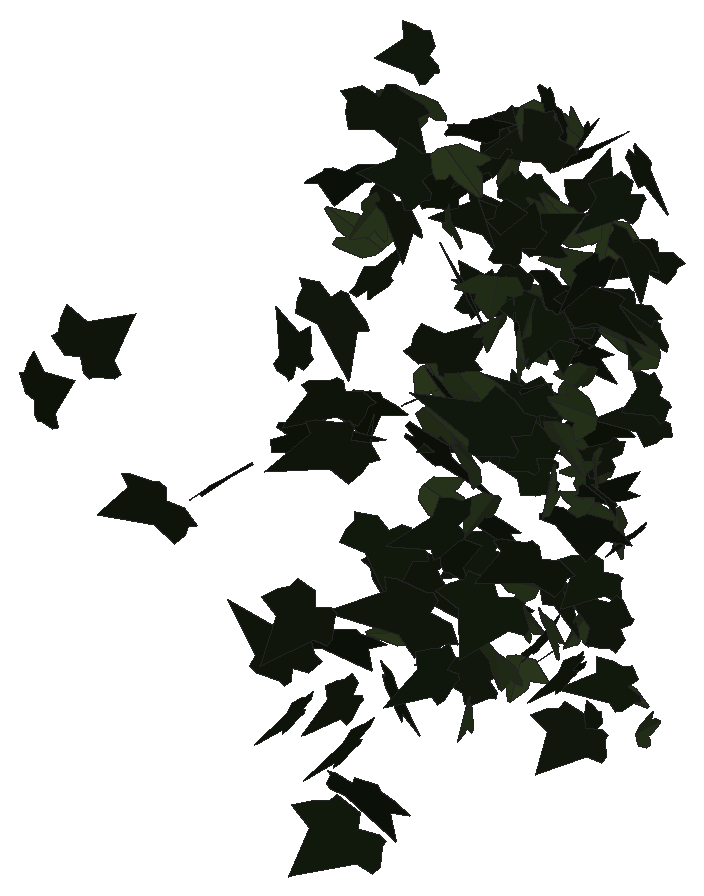
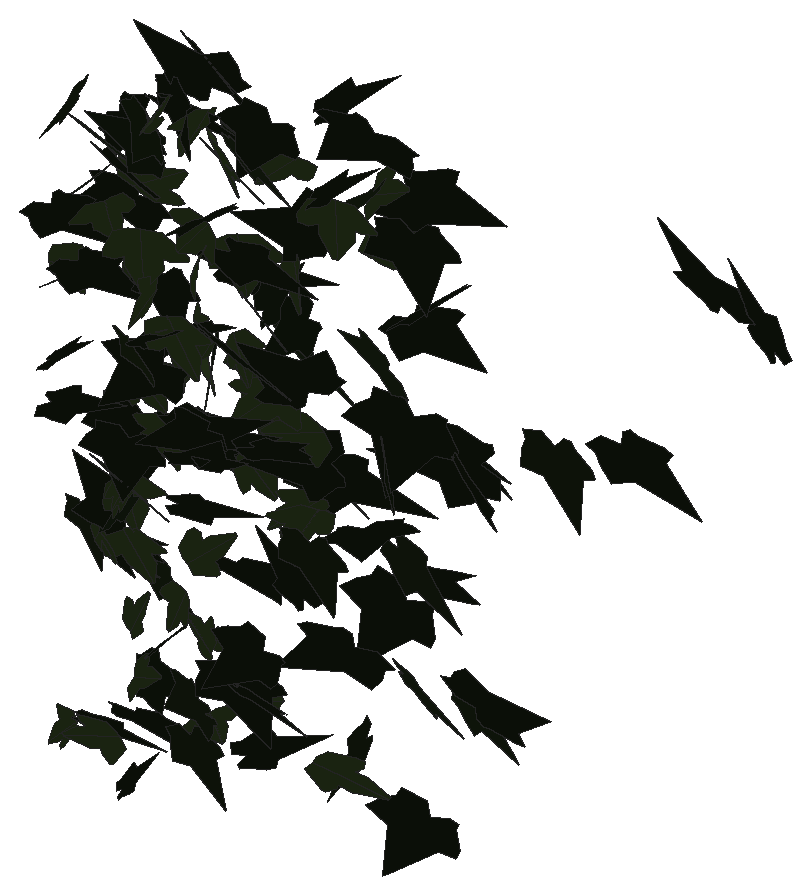
# SketchUp Ruby script. Lengths in inches.
U = 1.inch
M = Sketchup.active_model
def pt(a) = Geom::Point3d.new(a.map { |v| v * U })
def face(e, loops, mat)
  f = e.add_face(loops[0].map { |a| pt(a) })
  loops[1..].each { |l| e.add_face(l.map { |a| pt(a) }).erase! }
  f.material = f.back_material = mat if mat
  f
end
# faces: each face lists its corners as indices into pts; further lists are holes
def faces(e, pts, list, mat = nil) = list.each { |f| face(e, (f[0].is_a?(Array) ? f : [f]).map { |l| l.map { |i| pts[i] } }, mat) }
# xy, xz, yz: faces in a plane at the given z, y or x. An outline is a flat list of corners, or four numbers for a rectangle; further outlines are holes
def ring(l) = l.size == 4 ? [[l[0], l[1]], [l[2], l[1]], [l[2], l[3]], [l[0], l[3]]] : l.each_slice(2).to_a
def flat(e, list, mat, &to3) = list.each { |f| face(e, (f[0].is_a?(Array) ? f : [f]).map { |l| ring(l).map { |u, v| to3.(u, v) } }, mat) }
def xy(e, z, list, mat = nil) = flat(e, list, mat) { |x, y| [x, y, z] }
def xz(e, y, list, mat = nil) = flat(e, list, mat) { |x, z| [x, y, z] }
def yz(e, x, list, mat = nil) = flat(e, list, mat) { |y, z| [x, y, z] }
def lines(e, pts, list) = list.each { |a, b| e.add_line(pt(pts[a]), pt(pts[b])) }
# prism: a flat outline (further loops are holes) pulled along v
def prism(e, loops, v, mat = nil)
  f = face(e, loops, mat); d = Geom::Vector3d.new(v.map { |x| x * U })
  f.pushpull(f.normal.samedirection?(d) ? d.length : -d.length)
end
def box(e, o, s, mat = nil) = prism(e, [[o, [o[0] + s[0], o[1], o[2]], [o[0] + s[0], o[1] + s[1], o[2]], [o[0], o[1] + s[1], o[2]]]], [0, 0, s[2]], mat)
def at(x, y, z, deg = 0) = Geom::Transformation.translation(pt([x, y, z])) * Geom::Transformation.rotation(ORIGIN, Z_AXIS, deg.degrees)
def axes(o, x, y, z) = Geom::Transformation.new([*x, 0, *y, 0, *z, 0, *pt(o).to_a, 1])
def part(name) = M.definitions.add(name)
# library, detail: a bought-in or finely detailed component or shape, given as its bounding box
def library(name, o, s) = part(name).tap { |d| box(d.entities, o, s) }
def detail(e, o, s) = box(e.add_group.entities, o, s)
def put(e, d, t, mat = nil) = e.add_instance(d, t).tap { |i| i.material = mat if mat }
def group(e, t, mat = nil) = e.add_group.tap { |g| g.transformation = t; g.material = mat if mat }.entities
root = M.entities
M.materials.add("1026 AP 7946 SUNNY SIDE UP").color = [254, 231, 186]
M.materials.add("efeu1").color = [18, 25, 13]
M.materials.add("efeu2").color = [43, 57, 29]
c1 = part("ivyleaf_9")
p = [[1.54,2.16,1.25],[1.36,2.04,1.19],[-0.21,0.99,0.68],[-0.71,1.11,0.82],[-0.85,0.86,0.67],[-0.8,0.17,0.21],
  [-0.9,-0.01,0.1],[-0.67,-0.16,-0.02],[-0.08,-0.08,-0.05],[-0.03,-0.6,-0.4],[0.65,-0.88,-0.66],[0.83,-0.6,-0.49],
  [1.29,-0.42,-0.43],[1.8125,-0.07,-0.26],[1.21,0.44,0.15]]
faces(c1.entities,p,[[0,1,2,3,4,5,6,7,8,9,10,11,12,13,14]],"efeu1")
c2 = part("ivyleaf_10")
p = [[0,0.5,-0.03],[-0.0625,2.02,-0.43],[-0.19,2.01,-0.46],[-0.54,1.05,-0.29],[-0.52,0.625,-0.18],[-0.83,0.76,-0.28],
  [-1.16,0.64,-0.33],[-1.15,0.33,-0.24],[-0.77,-0.39,0.02],[-0.3,-0.51,0.16],[0.04,-0.48,0.23],[-0.02,2.01,-0.4375],
  [-0.06,2.01,-0.43],[0.04,-0.49,0.23],[0.67,-0.49,0.14],[1.38,0.36,-0.2],[1.375,0.51,-0.24],[0.81,0.65,-0.19],
  [0.62,0.59,-0.15],[0.6,1.09,-0.28],[0.5,1.23,-0.31]]
faces(c2.entities,p,[[0,1,2,3,4,5,6,7,8,9,10],[11,12,0,13,14,15,16,17,18,19,20]],"efeu2")
put(root,c1,axes([89.9,204.5625,274.55],[-0.05086,0.1436,0.39421],[0.18993,-0.34913,0.15144],[0.64039,0.11495,-0.01361]),"1026 AP 7946 SUNNY SIDE UP")
put(root,c1,axes([96.67,204.76,268.41],[-0.56224,-0.22577,0.12999],[-0.1429,-0.09664,-0.42919],[0.41356,-0.34033,0.02842]),"1026 AP 7946 SUNNY SIDE UP")
put(root,c1,axes([90.46,205.12,275.36],[-0.2526,0.22111,0.33746],[0.34026,-0.24042,0.2811],[0.55336,0.24877,-0.01881]),"1026 AP 7946 SUNNY SIDE UP")
put(root,c1,axes([95.93,205.48,275.42],[-0.08247,-0.01961,-0.43984],[-0.03894,-0.41267,0.01825],[-0.6967,0.02539,0.05105]),"1026 AP 7946 SUNNY SIDE UP")
put(root,c1,axes([94.96,205.73,271.71],[-0.65961,0.01646,-0.14293],[0.22051,-0.06256,-0.41322],[-0.0607,-0.40614,0.05205]),"1026 AP 7946 SUNNY SIDE UP")
put(root,c1,axes([91.76,205.69,272.69],[0.08639,0.01748,-0.39329],[-0.52238,-0.20149,-0.05868],[-0.34261,0.31163,-0.0097]),"1026 AP 7946 SUNNY SIDE UP")
put(root,c1,axes([95.93,205.72,269.49],[-0.3892,0.29505,-0.15727],[0.12168,-0.13481,-0.40107],[-0.54913,-0.23899,0.02259]),"1026 AP 7946 SUNNY SIDE UP")
put(root,c1,axes([95.94,205.67,268.62],[0.64221,0.04593,-0.10351],[-0.15486,-0.05156,-0.40657],[-0.09679,0.38721,-0.03628]),"1026 AP 7946 SUNNY SIDE UP")
put(root,c1,axes([97.34,206.36,271.05],[-0.56522,0.17945,-0.0836],[0.08926,-0.07116,-0.40401],[-0.32168,-0.33507,0.0348]),"1026 AP 7946 SUNNY SIDE UP")
put(root,c1,axes([92.29,206.66,272.89],[-0.04108,0.37676,-0.00245],[-0.00981,-0.00759,-0.40423],[-0.63961,-0.02408,0.00636]),"1026 AP 7946 SUNNY SIDE UP")
put(root,c1,axes([96.24,207.23,271.41],[-0.13267,-0.09029,-0.43018],[-0.4186,-0.31582,0.12329],[-0.55751,0.25862,0.00981]),"1026 AP 7946 SUNNY SIDE UP")
put(root,c1,axes([96.97,207.1,273.43],[-0.51236,0.28634,0.00295],[-0.03756,-0.02473,-0.44433],[-0.48462,-0.30081,0.03132]),"1026 AP 7946 SUNNY SIDE UP")
put(root,c1,axes([93.49,207.23,268.55],[-0.34705,0.22837,-0.13989],[0.1103,-0.12039,-0.32833],[-0.43542,-0.21252,0.02833]),"1026 AP 7946 SUNNY SIDE UP")
put(root,c1,axes([94.15,207.58,274.81],[0.0088,0.0949,-0.35614],[-0.09337,-0.32949,-0.10577],[-0.58181,0.05431,0.01159]),"1026 AP 7946 SUNNY SIDE UP")
put(root,c1,axes([94.1875,207.74,268.85],[-0.4841,0.14438,-0.13326],[0.15634,-0.09556,-0.34076],[-0.28571,-0.29692,0.03932]),"1026 AP 7946 SUNNY SIDE UP")
put(root,c1,axes([92.77,207.86,268.92],[-0.03693,0.09265,0.40653],[-0.46965,0.26332,-0.08235],[-0.46588,-0.27279,0.05079]),"1026 AP 7946 SUNNY SIDE UP")
put(root,c1,axes([97.27,208.14,274.87],[-0.26105,0.06281,0.39067],[-0.6115,0.06217,-0.1735],[-0.13941,-0.39031,0.02951]),"1026 AP 7946 SUNNY SIDE UP")
put(root,c1,axes([93.14,208.53,275.85],[0.01265,-0.41763,0.0121],[0.01009,-0.01664,-0.44737],[0.70944,0.00768,0.00615]),"1026 AP 7946 SUNNY SIDE UP")
put(root,c1,axes([92.58,208.15,273.2],[0.20135,0.20473,-0.32679],[0.17633,0.2919,0.25469],[0.60242,-0.15387,0.03468]),"1026 AP 7946 SUNNY SIDE UP")
put(root,c1,axes([94.32,208.6,271.7],[-0.22086,-0.34998,-0.07253],[0.04316,0.05795,-0.39891],[0.60217,-0.13252,0.00199]),"1026 AP 7946 SUNNY SIDE UP")
put(root,c1,axes([97.59,208.61,272.33],[0.09006,0.05264,-0.36108],[-0.31987,-0.28092,-0.08243],[-0.48456,0.19523,-0.0127]),"1026 AP 7946 SUNNY SIDE UP")
put(root,c1,axes([94.83,208.81,278.68],[-0.18583,-0.05194,0.37001],[-0.39925,-0.25789,-0.12461],[0.44038,-0.25572,0.04317]),"1026 AP 7946 SUNNY SIDE UP")
put(root,c2,axes([93.82,208.91,277.6875],[0.09185,0.12655,-0.34271],[-0.1388,-0.31176,-0.15034],[-0.57029,0.09626,-0.0186]),"1026 AP 7946 SUNNY SIDE UP")
put(root,c1,axes([97.28,208.51,278.39],[-0.1286,0.23965,0.34774],[-0.25371,0.28694,-0.26253],[-0.63193,-0.16397,0.03464]),"1026 AP 7946 SUNNY SIDE UP")
put(root,c1,axes([95.32,208.73,274.92],[0.51036,-0.15181,-0.09548],[-0.15401,0.01311,-0.35912],[0.25417,0.31277,-0.02589]),"1026 AP 7946 SUNNY SIDE UP")
put(root,c1,axes([93.33,208.72,273.95],[0.50052,0.24524,-0.09596],[-0.08811,-0.08235,-0.41053],[-0.43632,0.29795,-0.02718]),"1026 AP 7946 SUNNY SIDE UP")
put(root,c2,axes([95.7,209.06,268.54],[-0.06402,0.14317,-0.27763],[-0.0099,-0.26358,-0.15746],[-0.50553,-0.01297,0.03824]),"1026 AP 7946 SUNNY SIDE UP")
put(root,c1,axes([97.0625,208.84,278.33],[-0.1454,0.02222,0.3656],[0.55764,-0.09228,0.09343],[0.1611,0.33948,0.00657]),"1026 AP 7946 SUNNY SIDE UP")
put(root,c2,axes([97.64,208.79,273.29],[0.27612,-0.19541,0.23924],[-0.21075,0.18986,0.27404],[-0.46132,-0.2037,0.018]),"1026 AP 7946 SUNNY SIDE UP")
put(root,c1,axes([96.15,209.24,270.76],[-0.55963,-0.18525,-0.06897],[0.12781,-0.00824,-0.40227],[0.30601,-0.33535,0.04187]),"1026 AP 7946 SUNNY SIDE UP")
put(root,c2,axes([93.49,209.15,276.87],[0.21787,0.23196,0.23973],[-0.23915,-0.17284,0.27953],[0.48834,-0.18813,0.02994]),"1026 AP 7946 SUNNY SIDE UP")
put(root,c1,axes([97.92,209.09,270.07],[-0.3478,0.22407,-0.12194],[0.10476,-0.10147,-0.32566],[-0.41597,-0.2129,0.01994]),"1026 AP 7946 SUNNY SIDE UP")
put(root,c2,axes([95.93,209.27,272.5625],[-0.09551,-0.28271,0.16634],[-0.01972,-0.15957,-0.31027],[0.5503,-0.05478,0.01775]),"1026 AP 7946 SUNNY SIDE UP")
put(root,c1,axes([93.96,209.06,268.48],[0.39023,-0.18768,-0.21943],[-0.29069,0.10981,-0.31551],[0.36768,0.28601,-0.01655]),"1026 AP 7946 SUNNY SIDE UP")
put(root,c1,axes([93.85,209.41,277.61],[0.01709,-0.33166,0.16352],[0.00379,-0.15706,-0.35741],[0.62293,0.01005,-0.00231]),"1026 AP 7946 SUNNY SIDE UP")
put(root,c1,axes([93.56,208.97,272.98],[-0.00369,0.02646,0.36713],[0.06672,0.34036,-0.02312],[-0.57945,0.03902,-0.005]),"1026 AP 7946 SUNNY SIDE UP")
put(root,c2,axes([95.7,209.13,273.3],[0.14521,0.00768,-0.35048],[-0.30807,0.28287,-0.0397],[0.46291,0.18584,0.08352]),"1026 AP 7946 SUNNY SIDE UP")
put(root,c2,axes([95.61,209.35,274.3],[-0.5533,0.06345,-0.06679],[0.09517,-0.0415,-0.35467],[-0.11857,-0.32941,0.02697]),"1026 AP 7946 SUNNY SIDE UP")
put(root,c1,axes([94.37,209.42,273.16],[0.53961,-0.13917,0.17784],[0.23333,-0.10263,-0.37103],[0.28745,0.34455,-0.03267]),"1026 AP 7946 SUNNY SIDE UP")
put(root,c2,axes([96.14,209.375,269.52],[-0.44927,0.12539,0.06376],[-0.10725,0.00142,-0.31234],[-0.2085,-0.27092,0.02328]),"1026 AP 7946 SUNNY SIDE UP")
put(root,c2,axes([98.01,209.33,275.03],[0.12683,-0.10567,-0.33792],[-0.41907,0.19731,-0.13111],[0.37571,0.25576,-0.03217]),"1026 AP 7946 SUNNY SIDE UP")
put(root,c1,axes([98.07,209.61,277.82],[-0.10678,0.12233,-0.33205],[0.21847,-0.28402,-0.15108],[-0.52485,-0.14311,0.00467]),"1026 AP 7946 SUNNY SIDE UP")
put(root,c2,axes([94.6,209.54,273.65],[-0.30311,0.0262,-0.28964],[0.4287,-0.1048,-0.19052],[-0.17219,-0.30705,0.03551]),"1026 AP 7946 SUNNY SIDE UP")
put(root,c2,axes([94.74,209.34,272.32],[0.12672,0.19561,0.24277],[0.15526,0.20488,-0.22111],[-0.48065,0.11775,-0.00742]),"1026 AP 7946 SUNNY SIDE UP")
put(root,c2,axes([96.57,209.74,270.95],[-0.14064,-0.08574,-0.28912],[-0.26429,-0.21991,0.12333],[-0.39969,0.17558,0.02018]),"1026 AP 7946 SUNNY SIDE UP")
put(root,c1,axes([94.65,209.67,270.95],[-0.04228,0.06696,0.33181],[0.25665,-0.26977,0.07185],[0.47148,0.15285,-0.00935]),"1026 AP 7946 SUNNY SIDE UP")
put(root,c1,axes([97.74,209.52,272.77],[0.47019,0.17386,-0.17542],[-0.20979,-0.11446,-0.35043],[-0.35016,0.30202,-0.0256]),"1026 AP 7946 SUNNY SIDE UP")
put(root,c1,axes([92.58,209.61,277.68],[0.18937,0.31688,-0.12737],[-0.04681,-0.1207,-0.36106],[-0.57519,0.11415,-0.01255]),"1026 AP 7946 SUNNY SIDE UP")
put(root,c1,axes([91.6,209.48,273.69],[0.00277,0.107,0.37113],[-0.14281,0.3359,-0.10633],[-0.59676,-0.07989,0.02717]),"1026 AP 7946 SUNNY SIDE UP")
put(root,c1,axes([93.22,209.79,279.25],[-0.21276,-0.15737,-0.35862],[0.47717,0.1863,-0.20497],[0.40382,-0.30305,0.05326]),"1026 AP 7946 SUNNY SIDE UP")
put(root,c1,axes([93.66,209.73,270.44],[-0.06353,-0.10894,-0.37364],[0.40274,0.25785,-0.11026],[0.4692,-0.23607,0.04405]),"1026 AP 7946 SUNNY SIDE UP")
put(root,c2,axes([95.68,209.83,276.5],[-0.3676,-0.26586,0.02302],[0.00041,-0.03234,-0.36688],[0.45329,-0.21557,0.01899]),"1026 AP 7946 SUNNY SIDE UP")
put(root,c1,axes([95.17,210.01,273.39],[-0.42512,-0.12173,0.15658],[-0.1985,-0.09554,-0.29761],[0.25746,-0.27467,0.02908]),"1026 AP 7946 SUNNY SIDE UP")
put(root,c2,axes([96.75,209.9,270.25],[-0.33755,0.20561,-0.04061],[0.02098,-0.04438,-0.30596],[-0.35516,-0.19804,0.02052]),"1026 AP 7946 SUNNY SIDE UP")
put(root,c2,axes([94.98,209.93,274.3],[-0.45116,-0.04082,-0.18781],[0.30288,-0.02445,-0.28451],[0.03471,-0.31721,0.04158]),"1026 AP 7946 SUNNY SIDE UP")
put(root,c1,axes([98.28,209.89,270.6875],[-0.34006,-0.0315,-0.2572],[-0.40979,0.00624,0.21508],[-0.0261,0.31243,-0.02582]),"1026 AP 7946 SUNNY SIDE UP")
put(root,c1,axes([95.0625,210,275.79],[0.07827,-0.26839,0.22478],[-0.05049,0.21144,0.29444],[-0.57994,-0.05463,0.0047]),"1026 AP 7946 SUNNY SIDE UP")
put(root,c1,axes([97.31,210.16,268.24],[-0.55599,-0.09482,-0.03299],[0.06687,-0.03046,-0.36294],[0.15478,-0.32744,0.03832]),"1026 AP 7946 SUNNY SIDE UP")
put(root,c1,axes([94.43,209.85,274.56],[-0.15186,-0.02182,0.38516],[0.58265,0.10896,0.09989],[-0.18835,0.35464,-0.00156]),"1026 AP 7946 SUNNY SIDE UP")
put(root,c1,axes([92.92,209.84,275.45],[-0.21858,0.32063,0.00464],[0.01309,0.00293,0.36984],[0.54412,0.12873,-0.00703]),"1026 AP 7946 SUNNY SIDE UP")
put(root,c1,axes([97.51,209.99,276.8],[-0.031,-0.04797,-0.34205],[0.37144,0.23277,-0.04765],[0.4021,-0.21872,0.01765]),"1026 AP 7946 SUNNY SIDE UP")
put(root,c1,axes([95.11,210.29,268.38],[-0.1853,-0.02767,0.34281],[-0.46387,-0.17076,-0.11778],[0.28839,-0.29244,0.03082]),"1026 AP 7946 SUNNY SIDE UP")
put(root,c1,axes([96.22,210.17,273.18],[-0.10202,0.04202,0.33621],[-0.53578,0.013,-0.06646],[-0.03528,-0.31894,0.03705]),"1026 AP 7946 SUNNY SIDE UP")
put(root,c2,axes([95.95,210.23,269.91],[-0.11245,0.03581,0.28775],[0.40308,-0.12495,0.07887],[0.22065,0.24651,0.00257]),"1026 AP 7946 SUNNY SIDE UP")
put(root,c2,axes([94.54,210.07,278.46],[0.34845,0.17143,0.17417],[0.24281,0.07772,-0.28371],[-0.31609,0.24868,-0.02594]),"1026 AP 7946 SUNNY SIDE UP")
put(root,c1,axes([92.02,209.99,268.25],[0.46205,0.20669,0.00641],[0.0312,-0.01878,-0.36509],[-0.34952,0.27156,-0.02412]),"1026 AP 7946 SUNNY SIDE UP")
put(root,c1,axes([97.54,210.375,271.27],[-0.4258,-0.12235,0.01828],[-0.0091,-0.03142,-0.29793],[0.20989,-0.24956,0.02417]),"1026 AP 7946 SUNNY SIDE UP")
put(root,c1,axes([96.92,210.48,269.1875],[-0.23865,0.00163,-0.27866],[0.22385,-0.25464,-0.0815],[-0.38101,-0.15062,0.12666]),"1026 AP 7946 SUNNY SIDE UP")
put(root,c2,axes([93.56,210.39,268.74],[0.25756,-0.00409,-0.30195],[-0.47468,-0.04382,-0.161],[-0.06225,0.3172,-0.02162]),"1026 AP 7946 SUNNY SIDE UP")
put(root,c2,axes([95.76,210.4,268.83],[0.2476,0.22691,-0.11554],[-0.07647,-0.10262,-0.28969],[-0.42185,0.15178,-0.0153]),"1026 AP 7946 SUNNY SIDE UP")
put(root,c2,axes([95.21,210.44,275.31],[-0.03599,-0.29515,0.00399],[0.00823,-0.00794,-0.31685],[0.50112,-0.02107,0.00549]),"1026 AP 7946 SUNNY SIDE UP")
put(root,c1,axes([95.28,210.48,278.7],[-0.4624,0.18536,-0.13142],[0.13887,-0.10102,-0.35214],[-0.35337,-0.28224,0.03359]),"1026 AP 7946 SUNNY SIDE UP")
put(root,c1,axes([95.03,210.26,275.84],[-0.31884,0.0575,-0.24398],[-0.35355,0.09654,0.2105],[0.18757,0.27971,-0.01796]),"1026 AP 7946 SUNNY SIDE UP")
put(root,c1,axes([93.93,210.2,277.51],[0.08668,0.0548,0.38651],[0.5457,0.16465,-0.07328],[-0.2915,0.32453,-0.02226]),"1026 AP 7946 SUNNY SIDE UP")
put(root,c1,axes([94.77,210.28,279.08],[0.32802,0.23695,0.02958],[0.04082,0.01204,-0.32695],[-0.40232,0.19441,-0.00905]),"1026 AP 7946 SUNNY SIDE UP")
put(root,c2,axes([95.59,210.67,274.72],[-0.0155,-0.12035,-0.28507],[0.13581,-0.25565,0.11791],[-0.47456,-0.06923,0.04305]),"1026 AP 7946 SUNNY SIDE UP")
put(root,c1,axes([95.16,210.54,269.81],[0.27542,0.13577,-0.27266],[-0.30176,-0.18573,-0.22826],[-0.38935,0.23999,-0.01597]),"1026 AP 7946 SUNNY SIDE UP")
put(root,c2,axes([94.27,210.39,276.97],[-0.24896,0.14385,0.2828],[-0.34731,0.16487,-0.21698],[-0.37047,-0.25124,0.01337]),"1026 AP 7946 SUNNY SIDE UP")
put(root,c2,axes([95.74,210.78,275.52],[-0.00449,0.07249,-0.29341],[0.00177,-0.27502,-0.08146],[-0.48278,-0.00168,0.00243]),"1026 AP 7946 SUNNY SIDE UP")
put(root,c1,axes([95.9,210.65,273.7],[-0.05954,0.07388,0.3347],[-0.54263,0.01184,-0.04135],[-0.03454,-0.31341,0.07271]),"1026 AP 7946 SUNNY SIDE UP")
put(root,c1,axes([96.24,210.74,279.13],[-0.58732,0.03426,0.09539],[-0.15661,-0.04054,-0.36923],[-0.03882,-0.35485,0.04633]),"1026 AP 7946 SUNNY SIDE UP")
put(root,c2,axes([96.4,210.68,273.48],[-0.40622,0.11806,-0.1865],[0.22873,-0.11965,-0.28414],[-0.27722,-0.27172,0.03885]),"1026 AP 7946 SUNNY SIDE UP")
put(root,c2,axes([95.38,210.71,278.65],[0.36618,-0.27432,0.00927],[-0.01508,-0.02252,-0.37324],[0.46588,0.21488,-0.01937]),"1026 AP 7946 SUNNY SIDE UP")
put(root,c2,axes([96.83,210.64,277.52],[0.38652,0.10193,0.22142],[-0.33913,-0.05418,0.26499],[0.19136,-0.30189,0.02237]),"1026 AP 7946 SUNNY SIDE UP")
put(root,c1,axes([95.98,210.8,272.5],[-0.21174,-0.15937,-0.20935],[-0.23936,-0.13406,0.21368],[-0.35181,0.18713,-0.01938]),"1026 AP 7946 SUNNY SIDE UP")
put(root,c2,axes([98.28,210.69,275.7],[-0.05084,-0.00999,-0.31502],[-0.48974,0.05939,0.03012],[0.09868,0.28962,-0.01283]),"1026 AP 7946 SUNNY SIDE UP")
put(root,c1,axes([95.875,210.93,275.52],[-0.2776,-0.28196,0.02841],[-0.00127,-0.03445,-0.34899],[0.48138,-0.16269,0.01546]),"1026 AP 7946 SUNNY SIDE UP")
put(root,c1,axes([94.98,210.84,277.09],[-0.06873,-0.04438,-0.33046],[-0.38899,-0.20604,0.06114],[-0.35764,0.23262,-0.00299]),"1026 AP 7946 SUNNY SIDE UP")
put(root,c2,axes([95.74,210.58,275.11],[-0.03239,0.26016,0.22016],[-0.05192,0.20032,-0.27615],[-0.55698,-0.0338,0.01294]),"1026 AP 7946 SUNNY SIDE UP")
put(root,c1,axes([95.94,210.52,269.12],[-0.22212,0.21532,-0.19562],[-0.15612,0.16119,0.27195],[0.45652,0.15988,-0.00217]),"1026 AP 7946 SUNNY SIDE UP")
put(root,c1,axes([95.4,210.73,275.43],[0.1968,-0.11036,-0.3096],[-0.41487,0.15437,-0.16664],[0.31871,0.26909,-0.02575]),"1026 AP 7946 SUNNY SIDE UP")
put(root,c1,axes([95.75,210.79,273.28],[-0.45473,-0.10806,0.08392],[0.10646,0.05681,0.30855],[-0.20165,0.27367,-0.02634]),"1026 AP 7946 SUNNY SIDE UP")
put(root,c1,axes([96.1,210.93,270.28],[0.12907,-0.25634,-0.0605],[-0.03665,0.04903,-0.28548],[0.44289,0.07876,-0.00599]),"1026 AP 7946 SUNNY SIDE UP")
put(root,c1,axes([96.29,210.83,276.23],[0.3323,0.03605,-0.25173],[-0.38106,-0.0746,-0.21293],[-0.13602,0.29709,-0.01845]),"1026 AP 7946 SUNNY SIDE UP")
put(root,c1,axes([97.57,211.04,278.37],[-0.54169,0.04003,-0.10287],[0.13731,-0.10213,-0.33276],[-0.1125,-0.31738,0.08915]),"1026 AP 7946 SUNNY SIDE UP")
put(root,c2,axes([96.6,211.04,274.56],[-0.10362,-0.26764,0.15486],[-0.04542,-0.14581,-0.29586],[0.51729,-0.06641,0.00504]),"1026 AP 7946 SUNNY SIDE UP")
put(root,c1,axes([97.64,211.14,277.38],[0.01547,-0.3185,0.0866],[-0.01289,-0.08526,-0.34215],[0.55946,0.00684,-0.01028]),"1026 AP 7946 SUNNY SIDE UP")
put(root,c1,axes([95.74,210.87,268.68],[-0.13414,0.30246,-0.05992],[0.01299,-0.05991,-0.33541],[-0.52325,-0.07902,0.00703]),"1026 AP 7946 SUNNY SIDE UP")
put(root,c1,axes([95.625,210.73,273.84],[0.03917,0.10228,-0.28134],[0.02526,0.2642,0.11461],[0.48015,-0.02224,0.01692]),"1026 AP 7946 SUNNY SIDE UP")
put(root,c1,axes([96.79,211.15,267.625],[-0.05819,-0.0263,0.26494],[-0.22573,-0.20963,-0.04644],[0.35778,-0.13654,0.01379]),"1026 AP 7946 SUNNY SIDE UP")
put(root,c2,axes([96.61,211,276.78],[-0.49043,-0.18599,0.02466],[0.01358,-0.05889,-0.36415],[0.31838,-0.28399,0.05352]),"1026 AP 7946 SUNNY SIDE UP")
put(root,c1,axes([97.76,211.21,275.91],[-0.16872,-0.27771,0.12777],[0.02356,-0.1334,-0.31239],[0.51503,-0.08487,0.05614]),"1026 AP 7946 SUNNY SIDE UP")
put(root,c2,axes([95.5,211.01,277.4],[-0.40761,0.14252,-0.15008],[0.16509,-0.1114,-0.29723],[-0.29903,-0.25577,0.04048]),"1026 AP 7946 SUNNY SIDE UP")
put(root,c2,axes([96.53,211.16,269.59],[0.02973,0.1232,-0.26264],[-0.10664,-0.23916,-0.13585],[-0.45616,0.06394,0.01464]),"1026 AP 7946 SUNNY SIDE UP")
put(root,c1,axes([97.73,210.85,271.76],[-0.0519,0.26335,0.07578],[-0.01546,0.06674,-0.2829],[-0.46118,-0.03187,0.00096]),"1026 AP 7946 SUNNY SIDE UP")
put(root,c1,axes([95.1,211.09,278.8125],[-0.45829,0.08078,-0.11616],[0.15777,-0.06839,-0.30014],[-0.16882,-0.28321,0.03484]),"1026 AP 7946 SUNNY SIDE UP")
put(root,c1,axes([96.03,211.16,275.47],[-0.20019,-0.30435,-0.05158],[0.07199,0.03081,-0.3477],[0.51708,-0.12212,0.02844]),"1026 AP 7946 SUNNY SIDE UP")
put(root,c1,axes([97.58,211.17,276.17],[0.03599,0.01313,-0.32538],[-0.16059,-0.28945,-0.02448],[-0.49111,0.09561,-0.01584]),"1026 AP 7946 SUNNY SIDE UP")
put(root,c2,axes([95.52,210.94,279.23],[0.0616,0.32059,0.08789],[0.0272,0.07658,-0.34426],[-0.5594,0.03903,-0.00706]),"1026 AP 7946 SUNNY SIDE UP")
put(root,c2,axes([96.57,211.23,270.5],[-0.0256,-0.10998,-0.25706],[-0.06395,-0.23569,0.11553],[-0.4415,0.04052,-0.00183]),"1026 AP 7946 SUNNY SIDE UP")
put(root,c1,axes([95.28,211.1875,277.73],[0.00241,-0.34127,-0.03834],[0.03227,0.03139,-0.36435],[0.58087,-0.00033,0.0204]),"1026 AP 7946 SUNNY SIDE UP")
put(root,c2,axes([92.9375,211.05,278.59],[-0.53647,-0.06451,0.04077],[-0.05725,-0.02897,-0.34494],[0.11436,-0.31709,0.01858]),"1026 AP 7946 SUNNY SIDE UP")
put(root,c1,axes([96.03,210.99,279.56],[0.20517,-0.0542,-0.31024],[-0.49224,0.03032,-0.13546],[0.08351,0.31186,-0.03622]),"1026 AP 7946 SUNNY SIDE UP")
put(root,c2,axes([98.04,210.89,268.11],[0.04005,0.01079,0.27485],[-0.11473,0.24885,-0.00107],[-0.42059,-0.06685,0.02646]),"1026 AP 7946 SUNNY SIDE UP")
put(root,c1,axes([95.16,211,275.61],[-0.34567,0.21231,0.17849],[-0.24428,0.08726,-0.3111],[-0.3843,-0.24644,0.0372]),"1026 AP 7946 SUNNY SIDE UP")
put(root,c1,axes([98.01,211.33,274.47],[-0.16809,-0.13498,0.23522],[-0.17701,-0.19634,-0.18076],[0.40313,-0.14249,0.01871]),"1026 AP 7946 SUNNY SIDE UP")
put(root,c2,axes([96.48,210.9,275.9375],[-0.05383,0.13739,0.30885],[-0.14143,0.27446,-0.14684],[-0.52082,-0.08873,0.00795]),"1026 AP 7946 SUNNY SIDE UP")
put(root,c2,axes([96.73,211.18,272.6875],[-0.24806,-0.26525,0.04341],[-0.01594,-0.04502,-0.32452],[0.45615,-0.14582,0.01227]),"1026 AP 7946 SUNNY SIDE UP")
put(root,c2,axes([97.12,211.27,271.8],[0.29846,-0.12051,0.22431],[0.29488,-0.11994,-0.22987],[0.28863,0.24716,0.0029]),"1026 AP 7946 SUNNY SIDE UP")
put(root,c2,axes([95.91,211.15,275.62],[-0.47973,0.0059,0.18094],[-0.28563,-0.0414,-0.30037],[0.02754,-0.32664,0.03671]),"1026 AP 7946 SUNNY SIDE UP")
put(root,c1,axes([96.85,211.13,272.21],[0.37429,0.20497,0.02703],[-0.05479,0.00165,0.32137],[0.34574,-0.22164,0.02166]),"1026 AP 7946 SUNNY SIDE UP")
put(root,c1,axes([96.74,211.375,272.29],[0.27183,-0.21185,-0.14055],[0.15752,-0.09062,0.28243],[-0.39002,-0.18425,0.0161]),"1026 AP 7946 SUNNY SIDE UP")
put(root,c1,axes([97.36,211.26,268.6],[-0.41723,0.03124,0.14382],[-0.23276,-0.03442,-0.26127],[-0.01809,-0.27778,0.04457]),"1026 AP 7946 SUNNY SIDE UP")
put(root,c2,axes([96.68,211.23,271.86],[-0.45847,-0.00826,0.14999],[-0.22154,-0.09754,-0.27665],[0.08811,-0.28825,0.08483]),"1026 AP 7946 SUNNY SIDE UP")
put(root,c2,axes([93.33,211.1,273.35],[0.27593,0.26176,0.13353],[0.08478,0.11161,-0.3279],[-0.48235,0.16935,0.01875]),"1026 AP 7946 SUNNY SIDE UP")
put(root,c2,axes([96.24,211.3,278.95],[-0.13222,0.23831,0.16432],[0.01855,-0.15334,0.26408],[0.47799,0.07187,0.0352]),"1026 AP 7946 SUNNY SIDE UP")
put(root,c1,axes([96.1875,211.07,274.9],[0.50051,0.12556,0.05041],[0.09325,-0.01364,-0.34137],[-0.2066,0.29802,-0.03196]),"1026 AP 7946 SUNNY SIDE UP")
put(root,c1,axes([94.39,211.34,270.16],[-0.51346,0.03022,-0.01045],[0.00903,-0.04774,-0.32219],[-0.05336,-0.29885,0.04609]),"1026 AP 7946 SUNNY SIDE UP")
put(root,c2,axes([97.02,211.3,277.36],[0.26726,0.27686,-0.10956],[-0.09523,-0.08996,-0.3422],[-0.49412,0.16709,0.00669]),"1026 AP 7946 SUNNY SIDE UP")
put(root,c1,axes([96.79,211.09,277.91],[-0.42281,0.19828,0.02337],[0.04457,0.00213,0.34031],[0.33521,0.2498,-0.01577]),"1026 AP 7946 SUNNY SIDE UP")
put(root,c1,axes([97.61,211.26,278.99],[0.28762,-0.23345,-0.12926],[-0.15068,0.08055,-0.30673],[0.41744,0.18993,-0.02166]),"1026 AP 7946 SUNNY SIDE UP")
put(root,c2,axes([96.82,211.19,272.8],[-0.09425,0.29684,0.06909],[-0.09935,0.05001,-0.3186],[-0.50463,-0.06529,0.04982]),"1026 AP 7946 SUNNY SIDE UP")
put(root,c2,axes([95.47,211.13,276.72],[-0.11453,0.22602,-0.20495],[-0.06583,0.19096,0.25477],[0.50175,0.07665,-0.01335]),"1026 AP 7946 SUNNY SIDE UP")
put(root,c1,axes([96.68,211.2,273.51],[0.3031,0.20948,-0.10051],[-0.08549,-0.08383,-0.2954],[-0.38216,0.1849,-0.01363]),"1026 AP 7946 SUNNY SIDE UP")
put(root,c1,axes([97.87,211.45,277.15],[0.02178,0.04306,-0.31628],[-0.10931,-0.28891,-0.05201],[-0.49583,0.06558,-0.00243]),"1026 AP 7946 SUNNY SIDE UP")
put(root,c1,axes([94.1875,211.22,270.84],[0.52657,0.01607,0.00231],[0.0052,-0.02148,-0.33203],[-0.02699,0.30946,-0.01882]),"1026 AP 7946 SUNNY SIDE UP")
put(root,c1,axes([97.01,211.25,272.94],[-0.30623,0.19648,0.11186],[-0.16862,0.04563,-0.28177],[-0.33578,-0.20211,0.03949]),"1026 AP 7946 SUNNY SIDE UP")
put(root,c1,axes([97.8,211.51,273.9],[-0.07346,-0.13457,-0.25363],[-0.07307,-0.2317,0.14719],[-0.45408,0.05905,0.01735]),"1026 AP 7946 SUNNY SIDE UP")
put(root,c1,axes([96.27,211.15,278.55],[0.08644,0.29714,-0.07712],[0.01188,0.07581,0.32375],[0.52048,-0.05108,0.00542]),"1026 AP 7946 SUNNY SIDE UP")
put(root,c1,axes([92.76,211.59,279.16],[-0.19655,-0.08417,0.31246],[-0.29104,-0.24113,-0.15008],[0.42783,-0.2027,0.04146]),"1026 AP 7946 SUNNY SIDE UP")
put(root,c1,axes([93.24,211.21,272.95],[-0.00919,0.32749,0.00111],[-0.05885,-0.00379,-0.34873],[-0.55283,-0.00504,0.0371]),"1026 AP 7946 SUNNY SIDE UP")
put(root,c1,axes([96.39,211.12,278.86],[0.05723,0.20467,0.26106],[0.057,0.23886,-0.2187],[-0.53393,0.04743,0.00463]),"1026 AP 7946 SUNNY SIDE UP")
put(root,c2,axes([96.91,211.4,268.54],[-0.21701,-0.00161,-0.2497],[0.38533,-0.06195,-0.13361],[-0.09095,-0.25864,0.02974]),"1026 AP 7946 SUNNY SIDE UP")
put(root,c1,axes([96.55,211.1875,275.03],[-0.277,0.18532,-0.12833],[-0.144,0.08821,0.26553],[0.34832,0.18385,0.00772]),"1026 AP 7946 SUNNY SIDE UP")
